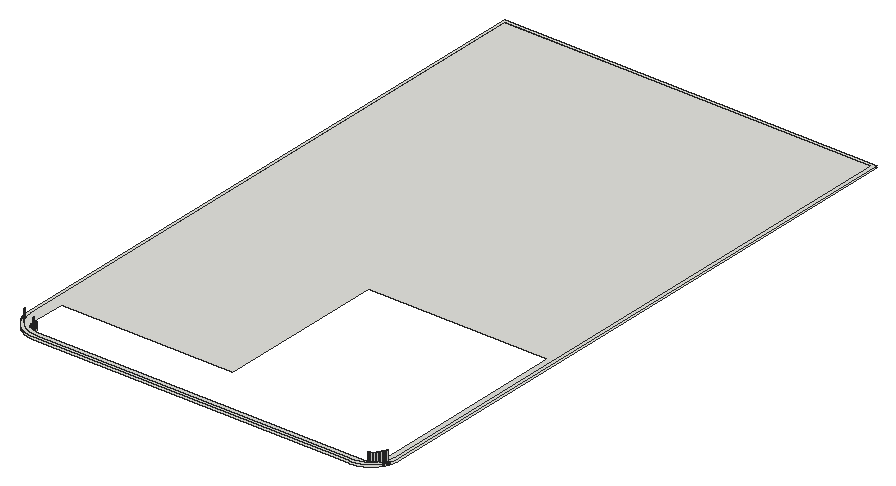
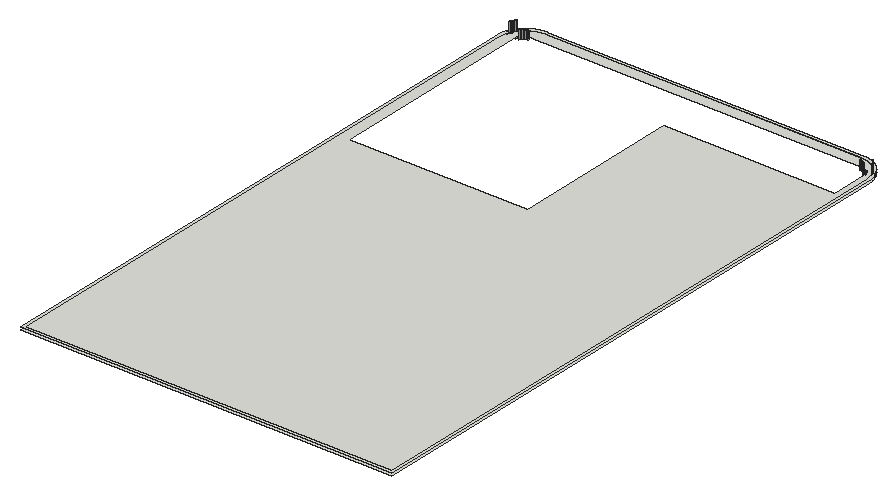
# SketchUp Ruby script. Lengths in inches.
U = 1.inch
M = Sketchup.active_model
def pt(a) = Geom::Point3d.new(a.map { |v| v * U })
def face(e, loops, mat)
  f = e.add_face(loops[0].map { |a| pt(a) })
  loops[1..].each { |l| e.add_face(l.map { |a| pt(a) }).erase! }
  f.material = f.back_material = mat if mat
  f
end
# faces: each face lists its corners as indices into pts; further lists are holes
def faces(e, pts, list, mat = nil) = list.each { |f| face(e, (f[0].is_a?(Array) ? f : [f]).map { |l| l.map { |i| pts[i] } }, mat) }
# xy, xz, yz: faces in a plane at the given z, y or x. An outline is a flat list of corners, or four numbers for a rectangle; further outlines are holes
def ring(l) = l.size == 4 ? [[l[0], l[1]], [l[2], l[1]], [l[2], l[3]], [l[0], l[3]]] : l.each_slice(2).to_a
def flat(e, list, mat, &to3) = list.each { |f| face(e, (f[0].is_a?(Array) ? f : [f]).map { |l| ring(l).map { |u, v| to3.(u, v) } }, mat) }
def xy(e, z, list, mat = nil) = flat(e, list, mat) { |x, y| [x, y, z] }
def xz(e, y, list, mat = nil) = flat(e, list, mat) { |x, z| [x, y, z] }
def yz(e, x, list, mat = nil) = flat(e, list, mat) { |y, z| [x, y, z] }
def lines(e, pts, list) = list.each { |a, b| e.add_line(pt(pts[a]), pt(pts[b])) }
# prism: a flat outline (further loops are holes) pulled along v
def prism(e, loops, v, mat = nil)
  f = face(e, loops, mat); d = Geom::Vector3d.new(v.map { |x| x * U })
  f.pushpull(f.normal.samedirection?(d) ? d.length : -d.length)
end
def box(e, o, s, mat = nil) = prism(e, [[o, [o[0] + s[0], o[1], o[2]], [o[0] + s[0], o[1] + s[1], o[2]], [o[0], o[1] + s[1], o[2]]]], [0, 0, s[2]], mat)
def at(x, y, z, deg = 0) = Geom::Transformation.translation(pt([x, y, z])) * Geom::Transformation.rotation(ORIGIN, Z_AXIS, deg.degrees)
def axes(o, x, y, z) = Geom::Transformation.new([*x, 0, *y, 0, *z, 0, *pt(o).to_a, 1])
def part(name) = M.definitions.add(name)
# library, detail: a bought-in or finely detailed component or shape, given as its bounding box
def library(name, o, s) = part(name).tap { |d| box(d.entities, o, s) }
def detail(e, o, s) = box(e.add_group.entities, o, s)
def put(e, d, t, mat = nil) = e.add_instance(d, t).tap { |i| i.material = mat if mat }
def group(e, t, mat = nil) = e.add_group.tap { |g| g.transformation = t; g.material = mat if mat }.entities
root = M.entities
xy(root,120,[[[23.87,144,23.56,144.01,22.92,144.03,22.61,144.05,22.29,144.07,21.98,144.1,21.66,144.13,21.35,144.17,21.03,144.21,20.72,144.25,20.4,144.3,19.78,144.4,19.16,144.52,18.54,144.66,18.23,144.74,17.93,144.82,17.62,144.9,17.02,145.08,16.71,145.17,16.41,145.27,16.11,145.375,15.82,145.48,15.52,145.59,15.23,145.71,14.93,145.83,14.35,146.07,14.0625,146.2,13.78,146.34,13.49,146.48,12.93,146.76,12.37,147.06,12.09,147.22,11.82,147.375,11.55,147.54,11.28,147.7,11.01,147.87,10.75,148.04,9.97,148.58,9.72,148.77,9.46,148.96,9.21,149.15,8.97,149.35,8.72,149.55,8.48,149.75,8.24,149.96,8,150.16,7.54,150.59,7.08,151.03,6.86,151.25,6.64,151.48,6.43,151.71,6.21,151.94,6,152.18,5.8,152.41,5.59,152.65,5.39,152.9,5.19,153.14,4.62,153.89,4.44,154.15,4.25,154.41,4.08,154.67,3.9,154.93,3.73,155.19,3.5625,155.46,3.4,155.73,3.08,156.27,2.78,156.83,2.64,157.1,2.49,157.39,2.36,157.67,2.22,157.95,1.96,158.53,1.72,159.11,1.5,159.69,1.28,160.29,1.18,160.58,1,161.18,0.91,161.49,0.82,161.79,0.74,162.09,0.67,162.4,0.6,162.7,0.46,163.32,0.41,163.625,0.35,163.9375,0.3,164.25,0.25,164.56,0.13,165.49,0.1,165.8,0.07,166.12,0.03,166.74,0.02,167.06,0.01,167.37,0,167.6875,0,672,314.45,672,314.45,167.37,314.43,167.06,314.42,166.74,314.38,166.12,314.35,165.8,314.29,165.18,314.25,164.87,314.2,164.56,314.16,164.25,314.1,163.9375,314.05,163.625,313.99,163.32,313.92,163.01,313.86,162.7,313.79,162.4,313.71,162.09,313.55,161.49,313.46,161.18,313.37,160.88,313.27,160.58,313.17,160.29,313.07,159.99,312.96,159.69,312.85,159.4,312.49,158.53,312.23,157.95,312.1,157.67,311.96,157.39,311.82,157.1,311.67,156.83,311.37,156.27,310.89,155.46,310.72,155.19,310.55,154.93,310.2,154.41,310.02,154.15,309.83,153.89,309.65,153.64,309.45,153.39,309.26,153.14,309.0625,152.9,308.86,152.65,308.66,152.41,308.45,152.18,308.24,151.94,308.03,151.71,307.8125,151.48,307.59,151.25,307.37,151.03,307.14,150.81,306.92,150.59,306.68,150.375,306.45,150.16,306.21,149.96,305.97,149.75,305.49,149.35,305.24,149.15,304.74,148.77,304.48,148.58,304.23,148.4,303.97,148.22,303.7,148.04,303.4375,147.87,303.17,147.7,302.9,147.54,302.63,147.375,302.36,147.22,302.08,147.06,301.81,146.91,301.53,146.76,301.25,146.62,300.96,146.48,300.68,146.34,300.39,146.2,300.1,146.07,299.8125,145.95,299.52,145.83,299.23,145.71,298.93,145.59,298.64,145.48,298.04,145.27,297.74,145.17,297.4375,145.08,297.13,144.99,296.83,144.9,296.53,144.82,295.91,144.66,295.29,144.52,294.67,144.4,293.74,144.25,293.42,144.21,293.11,144.17,292.79,144.13,292.48,144.1,292.16,144.07,291.85,144.05,291.53,144.03,291.21,144.02,290.9,144.01,290.58,144],[17.82,153,296.45,153,297.63,153.08,298.78,153.31,299.9,153.69,300.95,154.21,301.93,154.86,302.82,155.64,303.59,156.52,304.25,157.5,304.77,158.56,305.15,159.67,305.375,160.83,305.45,162,305.45,336,154.05,336,154.05,192,9,192,9,161.82,9.01,161.65,9.03,161.29,9.04,161.12,9.0625,160.94,9.08,160.77,9.11,160.59,9.14,160.42,9.17,160.24,9.29,159.73,9.44,159.22,9.56,158.88,9.62,158.72,9.69,158.56,9.75,158.39,9.83,158.23,9.9,158.07,9.98,157.91,10.0625,157.76,10.15,157.6,10.42,157.15,10.62,156.85,10.82,156.57,11.04,156.29,11.16,156.15,11.27,156.02,11.51,155.76,11.64,155.64,11.76,155.51,12.02,155.27,12.15,155.16,12.29,155.04,12.57,154.82,12.85,154.62,13.15,154.42,13.6,154.15,13.76,154.0625,13.91,153.98,14.07,153.9,14.23,153.83,14.39,153.75,14.56,153.69,14.72,153.62,14.88,153.56,15.22,153.44,15.73,153.29,16.24,153.17,16.42,153.14,16.59,153.11,16.77,153.08,16.94,153.0625,17.12,153.04,17.29,153.03,17.65,153.01]]])
xy(root,122,[[[23.87,144,290.58,144,290.9,144.01,291.21,144.02,291.53,144.03,291.85,144.05,292.16,144.07,292.48,144.1,292.79,144.13,293.11,144.17,293.42,144.21,293.74,144.25,294.67,144.4,295.29,144.52,295.91,144.66,296.53,144.82,296.83,144.9,297.13,144.99,297.4375,145.08,297.74,145.17,298.04,145.27,298.64,145.48,298.93,145.59,299.23,145.71,299.52,145.83,299.8125,145.95,300.1,146.07,300.39,146.2,300.68,146.34,300.96,146.48,301.25,146.62,301.53,146.76,301.81,146.91,302.08,147.06,302.36,147.22,302.63,147.375,302.9,147.54,303.17,147.7,303.4375,147.87,303.7,148.04,303.97,148.22,304.23,148.4,304.48,148.58,304.74,148.77,305.24,149.15,305.49,149.35,305.97,149.75,306.21,149.96,306.45,150.16,306.68,150.375,306.92,150.59,307.14,150.81,307.37,151.03,307.59,151.25,307.8125,151.48,308.03,151.71,308.24,151.94,308.45,152.18,308.66,152.41,308.86,152.65,309.0625,152.9,309.26,153.14,309.45,153.39,309.65,153.64,309.83,153.89,310.02,154.15,310.2,154.41,310.55,154.93,310.72,155.19,310.89,155.46,311.37,156.27,311.67,156.83,311.82,157.1,311.96,157.39,312.1,157.67,312.23,157.95,312.49,158.53,312.85,159.4,312.96,159.69,313.07,159.99,313.17,160.29,313.27,160.58,313.37,160.88,313.46,161.18,313.55,161.49,313.71,162.09,313.79,162.4,313.86,162.7,313.92,163.01,313.99,163.32,314.05,163.625,314.1,163.9375,314.16,164.25,314.2,164.56,314.25,164.87,314.29,165.18,314.35,165.8,314.38,166.12,314.42,166.74,314.43,167.06,314.45,167.37,314.45,672,0,672,0,167.6875,0.01,167.37,0.02,167.06,0.03,166.74,0.07,166.12,0.1,165.8,0.13,165.49,0.25,164.56,0.3,164.25,0.35,163.9375,0.41,163.625,0.46,163.32,0.6,162.7,0.67,162.4,0.74,162.09,0.82,161.79,0.91,161.49,1,161.18,1.18,160.58,1.28,160.29,1.5,159.69,1.72,159.11,1.96,158.53,2.22,157.95,2.36,157.67,2.49,157.39,2.64,157.1,2.78,156.83,3.08,156.27,3.4,155.73,3.5625,155.46,3.73,155.19,3.9,154.93,4.08,154.67,4.25,154.41,4.44,154.15,4.62,153.89,5.19,153.14,5.39,152.9,5.59,152.65,5.8,152.41,6,152.18,6.21,151.94,6.43,151.71,6.64,151.48,6.86,151.25,7.08,151.03,7.54,150.59,8,150.16,8.24,149.96,8.48,149.75,8.72,149.55,8.97,149.35,9.21,149.15,9.46,148.96,9.72,148.77,9.97,148.58,10.75,148.04,11.01,147.87,11.28,147.7,11.55,147.54,11.82,147.375,12.09,147.22,12.37,147.06,12.93,146.76,13.49,146.48,13.78,146.34,14.0625,146.2,14.35,146.07,14.93,145.83,15.23,145.71,15.52,145.59,15.82,145.48,16.11,145.375,16.41,145.27,16.71,145.17,17.02,145.08,17.62,144.9,17.93,144.82,18.23,144.74,18.54,144.66,19.16,144.52,19.78,144.4,20.4,144.3,20.72,144.25,21.03,144.21,21.35,144.17,21.66,144.13,21.98,144.1,22.29,144.07,22.61,144.05,22.92,144.03,23.56,144.01],[23.9,146,23.03,146.03,22.16,146.09,21.58,146.15,21.29,146.1875,21.01,146.23,20.72,146.27,20.43,146.32,20.15,146.37,19.86,146.42,19.3,146.54,19.01,146.61,18.45,146.75,17.61,146.99,17.34,147.08,17.0625,147.17,16.79,147.26,16.51,147.36,16.24,147.46,15.97,147.57,15.7,147.67,15.4375,147.79,15.17,147.9,14.91,148.02,14.64,148.14,13.86,148.53,13.61,148.67,13.35,148.81,12.85,149.09,12.6,149.24,12.36,149.39,12.11,149.55,11.39,150.03,11.16,150.2,10.92,150.37,10.69,150.55,10.46,150.72,10.23,150.9,10.01,151.09,9.79,151.27,9.35,151.65,9.14,151.84,8.51,152.44,7.71,153.28,7.52,153.49,7.14,153.93,6.96,154.15,6.42,154.84,6.08,155.3,5.92,155.54,5.75,155.78,5.59,156.02,5.4375,156.26,5.28,156.51,5.13,156.75,4.99,157,4.84,157.25,4.7,157.5,4.57,157.76,4.43,158.01,4.3,158.27,4.18,158.53,4.05,158.79,3.93,159.05,3.82,159.32,3.7,159.58,3.59,159.85,3.19,160.93,3.1,161.2,3.01,161.48,2.93,161.75,2.77,162.31,2.7,162.58,2.63,162.86,2.5625,163.14,2.5,163.43,2.44,163.71,2.34,164.27,2.29,164.56,2.25,164.84,2.21,165.13,2.17,165.41,2.11,165.99,2.08,166.27,2.0625,166.5625,2.05,166.85,2.03,167.14,2.02,167.42,2.02,670,312.4375,670,312.4375,167.71,312.43,167.42,312.42,167.14,312.41,166.85,312.39,166.5625,312.37,166.27,312.34,165.99,312.32,165.7,312.28,165.41,312.25,165.13,312.21,164.84,312.16,164.56,312.12,164.27,312.07,163.99,311.95,163.43,311.89,163.14,311.83,162.86,311.76,162.58,311.68,162.31,311.61,162.03,311.52,161.75,311.44,161.48,311.35,161.2,311.17,160.66,311.07,160.39,310.96,160.12,310.86,159.85,310.75,159.58,310.64,159.32,310.52,159.05,310.28,158.53,310.02,158.01,309.89,157.76,309.75,157.5,309.47,157,309.32,156.75,309.17,156.51,309.02,156.26,308.54,155.54,308.37,155.3,307.86,154.61,307.5,154.15,307.125,153.71,306.94,153.49,306.74,153.28,306.55,153.07,306.15,152.65,305.74,152.24,305.32,151.84,304.66,151.27,304.44,151.09,304.22,150.9,303.99,150.72,303.76,150.55,303.53,150.37,303.3,150.2,303.0625,150.03,302.82,149.87,302.1,149.39,301.6,149.09,301.1,148.81,300.84,148.67,300.59,148.53,299.81,148.14,299.55,148.02,299.28,147.9,299.02,147.79,298.75,147.67,298.48,147.57,298.21,147.46,297.9375,147.36,297.67,147.26,297.39,147.17,297.12,147.08,296.84,146.99,296.5625,146.91,296.28,146.83,296,146.75,295.16,146.54,294.59,146.42,294.31,146.37,293.73,146.27,293.45,146.23,293.16,146.1875,292.87,146.15,292.29,146.09,291.71,146.05,291.43,146.03,290.85,146.01,290.55,146]]])
p = [[302.82,155.64,120],[301.93,154.86,120],[301.93,154.86,119],[302.82,155.64,119],[12.29,155.04,120],[12.15,155.16,120],
  [12.15,155.16,119],[12.29,155.04,119],[17.04,155.07,126],[17.18,155.05,126],[17.18,155.05,119],[17.04,155.07,119],
  [17.3125,155.03,126],[17.3125,155.03,119],[16.5,155.16,126],[16.63,155.13,126],[16.63,155.13,119],[16.5,155.16,119],
  [16.77,155.11,126],[16.77,155.11,119],[16.9,155.09,126],[16.9,155.09,119],[297.37,155.06,126],[298.27,155.24,126],
  [298.27,155.24,119],[297.37,155.06,119],[12.02,155.27,120],[12.02,155.27,119],[16.1,155.26,126],[16.23,155.23,126],
  [16.23,155.23,119],[16.1,155.26,119],[16.37,155.19,126],[16.37,155.19,119],[299.13,155.53,126],[299.13,155.53,119],
  [11.89,155.39,120],[11.89,155.39,119],[15.71,155.39,126],[15.84,155.34,126],[15.84,155.34,119],[15.71,155.39,119],
  [15.97,155.3,126],[15.97,155.3,119],[11.76,155.51,120],[11.76,155.51,119],[15.45,155.48,126],[15.58,155.43,126],
  [15.58,155.43,119],[15.45,155.48,119],[11.64,155.64,120],[11.64,155.64,119],[15.19,155.59,126],[15.32,155.53,126],
  [15.32,155.53,119],[15.19,155.59,119],[299.95,155.9375,126],[299.95,155.9375,119],[11.51,155.76,120],[11.51,155.76,119],
  [14.95,155.7,126],[15.07,155.64,126],[15.07,155.64,119],[14.95,155.7,119],[303.59,156.52,120],[303.59,156.52,119],
  [14.82,155.76,126],[14.82,155.76,119],[11.39,155.89,120],[11.39,155.89,119],[14.58,155.89,126],[14.7,155.83,126],
  [14.7,155.83,119],[14.58,155.89,119],[11.27,156.02,120],[11.27,156.02,119],[14.46,155.96,126],[14.46,155.96,119],
  [300.71,156.45,126],[300.71,156.45,119],[11.16,156.15,120],[11.16,156.15,119],[14.23,156.1,126],[14.34,156.03,126],
  [14.34,156.03,119],[14.23,156.1,119],[14.11,156.18,126],[14.11,156.18,119],[11.04,156.29,120],[11.04,156.29,119],
  [14,156.26,126],[14,156.26,119],[10.93,156.43,120],[10.93,156.43,119],[13.78,156.42,126],[13.89,156.34,126],
  [13.89,156.34,119],[13.78,156.42,119],[10.82,156.57,120],[10.82,156.57,119],[13.67,156.5,126],[13.67,156.5,119],
  [301.4,157.05,126],[301.4,157.05,119],[13.56,156.59,126],[13.56,156.59,119],[304.25,157.5,120],[304.25,157.5,119],
  [10.72,156.71,120],[10.72,156.71,119],[13.45,156.68,126],[13.45,156.68,119],[10.62,156.85,120],[10.62,156.85,119],
  [13.35,156.77,126],[13.35,156.77,119],[13.25,156.86,126],[13.25,156.86,119],[10.52,157,120],[10.52,157,119],
  [13.15,156.95,126],[13.15,156.95,119],[10.42,157.15,120],[10.42,157.15,119],[13.05,157.05,126],[13.05,157.05,119],
  [10.33,157.3,120],[10.33,157.3,119],[12.86,157.25,126],[12.95,157.15,126],[12.95,157.15,119],[12.86,157.25,119],
  [302.01,157.74,126],[302.01,157.74,119],[12.77,157.35,126],[12.77,157.35,119],[10.24,157.45,120],[10.24,157.45,119],
  [10.15,157.6,120],[10.15,157.6,119],[12.68,157.45,126],[12.68,157.45,119],[12.59,157.56,126],[12.59,157.56,119],
  [304.77,158.56,120],[304.77,158.56,119],[10.0625,157.76,120],[10.0625,157.76,119],[12.5,157.67,126],[12.5,157.67,119],
  [12.42,157.78,126],[12.42,157.78,119],[302.52,158.5,126],[302.52,158.5,119],[9.98,157.91,120],[9.98,157.91,119],
  [12.34,157.89,126],[12.34,157.89,119],[9.9,158.07,120],[9.9,158.07,119],[12.26,158,126],[12.26,158,119],
  [12.18,158.11,126],[12.18,158.11,119],[9.83,158.23,120],[9.83,158.23,119],[12.1,158.23,126],[12.1,158.23,119],
  [9.75,158.39,120],[9.75,158.39,119],[12.03,158.34,126],[12.03,158.34,119],[11.96,158.46,126],[11.96,158.46,119],
  [9.69,158.56,120],[9.69,158.56,119],[11.89,158.58,126],[11.89,158.58,119],[302.92,159.32,126],[302.92,159.32,119],
  [9.62,158.72,120],[9.62,158.72,119],[11.83,158.7,126],[11.83,158.7,119],[305.15,159.67,120],[305.15,159.67,119],
  [9.56,158.88,120],[9.56,158.88,119],[11.76,158.82,126],[11.76,158.82,119],[11.7,158.95,126],[11.7,158.95,119],
  [9.5,159.05,120],[9.5,159.05,119],[11.64,159.07,126],[11.64,159.07,119],[9.44,159.22,120],[9.44,159.22,119],
  [11.59,159.19,126],[11.59,159.19,119],[9.39,159.39,120],[9.39,159.39,119],[11.53,159.32,126],[11.53,159.32,119],
  [11.48,159.45,126],[11.48,159.45,119],[9.34,159.56,120],[9.34,159.56,119],[11.43,159.58,126],[11.43,159.58,119],
  [3.73,155.19,120],[3.9,154.93,120],[3.9,154.93,122],[3.73,155.19,122],[310.55,154.93,120],[310.72,155.19,120],
  [310.72,155.19,122],[310.55,154.93,122],[3.5625,155.46,120],[3.5625,155.46,122],[310.89,155.46,120],[310.89,155.46,122],
  [3.4,155.73,120],[3.4,155.73,122],[311.05,155.73,120],[311.05,155.73,122],[3.24,156,120],[3.24,156,122],
  [311.21,156,120],[311.21,156,122],[3.08,156.27,120],[3.08,156.27,122],[311.37,156.27,120],[311.37,156.27,122],
  [2.93,156.55,120],[2.93,156.55,122],[311.52,156.55,120],[311.52,156.55,122],[2.78,156.83,120],[2.78,156.83,122],
  [311.67,156.83,120],[311.67,156.83,122],[2.64,157.1,120],[2.64,157.1,122],[311.82,157.1,120],[311.82,157.1,122],
  [2.49,157.39,120],[2.49,157.39,122],[311.96,157.39,120],[311.96,157.39,122],[2.36,157.67,120],[2.36,157.67,122],
  [312.1,157.67,120],[312.1,157.67,122],[2.22,157.95,120],[2.22,157.95,122],[312.23,157.95,120],[312.23,157.95,122],
  [2.09,158.24,120],[2.09,158.24,122],[312.36,158.24,120],[312.36,158.24,122],[1.96,158.53,120],[1.96,158.53,122],
  [312.49,158.53,120],[312.49,158.53,122],[1.84,158.82,120],[1.84,158.82,122],[312.61,158.82,120],[312.61,158.82,122],
  [1.72,159.11,120],[1.72,159.11,122],[312.73,159.11,120],[312.73,159.11,122],[1.61,159.4,120],[1.61,159.4,122],
  [312.85,159.4,120],[312.85,159.4,122],[1.5,159.69,120],[1.5,159.69,122],[312.96,159.69,120],[312.96,159.69,122],
  [6.08,155.3,122],[6.25,155.07,122],[6.25,155.07,130],[6.08,155.3,130],[308.2,155.07,122],[308.37,155.3,122],
  [308.37,155.3,130],[308.2,155.07,130],[5.92,155.54,122],[5.92,155.54,130],[308.54,155.54,122],[308.54,155.54,130],
  [5.75,155.78,122],[5.75,155.78,130],[308.7,155.78,122],[308.7,155.78,130],[5.59,156.02,122],[5.59,156.02,130],
  [308.86,156.02,122],[308.86,156.02,130],[5.4375,156.26,122],[5.4375,156.26,130],[309.02,156.26,122],[309.02,156.26,130],
  [5.28,156.51,122],[5.28,156.51,130],[309.17,156.51,122],[309.17,156.51,130],[5.13,156.75,122],[5.13,156.75,130],
  [309.32,156.75,122],[309.32,156.75,130],[4.99,157,122],[4.99,157,130],[309.47,157,122],[309.47,157,130],
  [4.84,157.25,122],[4.84,157.25,130],[309.61,157.25,122],[309.61,157.25,130],[4.7,157.5,122],[4.7,157.5,130],
  [309.75,157.5,122],[309.75,157.5,130],[4.57,157.76,122],[4.57,157.76,130],[309.89,157.76,122],[309.89,157.76,130],
  [4.43,158.01,122],[4.43,158.01,130],[310.02,158.01,122],[310.02,158.01,130],[4.3,158.27,122],[4.3,158.27,130],
  [310.15,158.27,122],[310.15,158.27,130],[4.18,158.53,122],[4.18,158.53,130],[310.28,158.53,122],[310.28,158.53,130],
  [4.05,158.79,122],[4.05,158.79,130],[310.4,158.79,122],[310.4,158.79,130],[3.93,159.05,122],[3.93,159.05,130],
  [310.52,159.05,122],[310.52,159.05,130],[3.82,159.32,122],[3.82,159.32,130],[310.64,159.32,122],[310.64,159.32,130],
  [3.7,159.58,122],[3.7,159.58,130],[310.75,159.58,122],[310.75,159.58,130]]
faces(root,p,[[0,1,2,3],[4,5,6,7],[8,9,10,11],[9,12,13,10],[14,15,16,17],[15,18,19,16],[18,20,21,19],[20,8,11,21],
  [22,23,24,25],[5,26,27,6],[28,29,30,31],[29,32,33,30],[32,14,17,33],[23,34,35,24],[26,36,37,27],[38,39,40,41],
  [39,42,43,40],[42,28,31,43],[36,44,45,37],[46,47,48,49],[47,38,41,48],[44,50,51,45],[52,53,54,55],[53,46,49,54],
  [34,56,57,35],[50,58,59,51],[60,61,62,63],[61,52,55,62],[64,0,3,65],[66,60,63,67],[58,68,69,59],[70,71,72,73],
  [71,66,67,72],[68,74,75,69],[76,70,73,77],[56,78,79,57],[74,80,81,75],[82,83,84,85],[83,76,77,84],[86,82,85,87],
  [80,88,89,81],[90,86,87,91],[88,92,93,89],[94,95,96,97],[95,90,91,96],[92,98,99,93],[100,94,97,101],[78,102,103,79],
  [104,100,101,105],[106,64,65,107],[98,108,109,99],[110,104,105,111],[108,112,113,109],[114,110,111,115],[116,114,115,117],[112,118,119,113],
  [120,116,117,121],[118,122,123,119],[124,120,121,125],[122,126,127,123],[128,129,130,131],[129,124,125,130],[102,132,133,103],[134,128,131,135],
  [126,136,137,127],[136,138,139,137],[140,134,135,141],[142,140,141,143],[144,106,107,145],[138,146,147,139],[148,142,143,149],[150,148,149,151],
  [132,152,153,133],[146,154,155,147],[156,150,151,157],[154,158,159,155],[160,156,157,161],[162,160,161,163],[158,164,165,159],[166,162,163,167],
  [164,168,169,165],[170,166,167,171],[172,170,171,173],[168,174,175,169],[176,172,173,177],[152,178,179,153],[174,180,181,175],[182,176,177,183],
  [184,144,145,185],[180,186,187,181],[188,182,183,189],[190,188,189,191],[186,192,193,187],[194,190,191,195],[192,196,197,193],[198,194,195,199],
  [196,200,201,197],[202,198,199,203],[204,202,203,205],[200,206,207,201],[208,204,205,209],[210,211,212,213],[214,215,216,217],[218,210,213,219],
  [215,220,221,216],[222,218,219,223],[220,224,225,221],[226,222,223,227],[224,228,229,225],[230,226,227,231],[228,232,233,229],[234,230,231,235],
  [232,236,237,233],[238,234,235,239],[236,240,241,237],[242,238,239,243],[240,244,245,241],[246,242,243,247],[244,248,249,245],[250,246,247,251],
  [248,252,253,249],[254,250,251,255],[252,256,257,253],[258,254,255,259],[256,260,261,257],[262,258,259,263],[260,264,265,261],[266,262,263,267],
  [264,268,269,265],[270,266,267,271],[268,272,273,269],[274,270,271,275],[272,276,277,273],[278,274,275,279],[276,280,281,277],[282,283,284,285],
  [286,287,288,289],[290,282,285,291],[287,292,293,288],[294,290,291,295],[292,296,297,293],[298,294,295,299],[296,300,301,297],[302,298,299,303],
  [300,304,305,301],[306,302,303,307],[304,308,309,305],[310,306,307,311],[308,312,313,309],[314,310,311,315],[312,316,317,313],[318,314,315,319],
  [316,320,321,317],[322,318,319,323],[320,324,325,321],[326,322,323,327],[324,328,329,325],[330,326,327,331],[328,332,333,329],[334,330,331,335],
  [332,336,337,333],[338,334,335,339],[336,340,341,337],[342,338,339,343],[340,344,345,341],[346,342,343,347],[344,348,349,345],[350,346,347,351],
  [348,352,353,349],[354,350,351,355],[352,356,357,353]])
